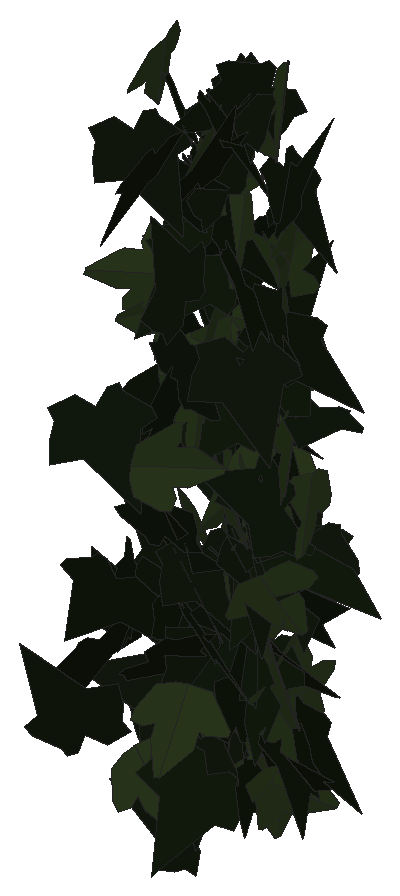
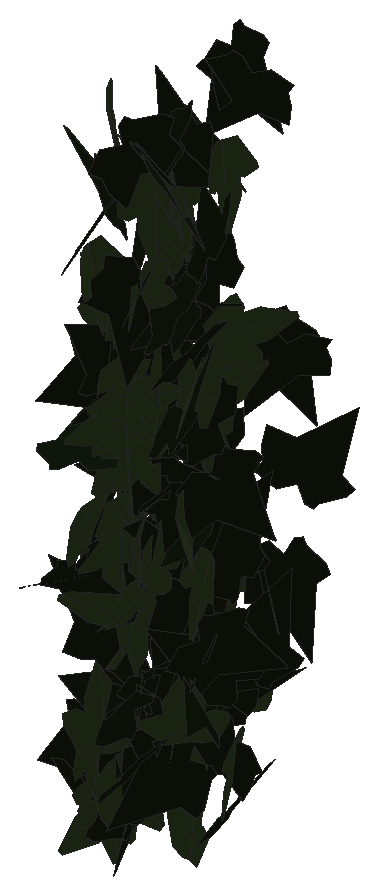
# SketchUp Ruby script. Lengths in inches.
U = 1.inch
M = Sketchup.active_model
def pt(a) = Geom::Point3d.new(a.map { |v| v * U })
def face(e, loops, mat)
  f = e.add_face(loops[0].map { |a| pt(a) })
  loops[1..].each { |l| e.add_face(l.map { |a| pt(a) }).erase! }
  f.material = f.back_material = mat if mat
  f
end
# faces: each face lists its corners as indices into pts; further lists are holes
def faces(e, pts, list, mat = nil) = list.each { |f| face(e, (f[0].is_a?(Array) ? f : [f]).map { |l| l.map { |i| pts[i] } }, mat) }
# xy, xz, yz: faces in a plane at the given z, y or x. An outline is a flat list of corners, or four numbers for a rectangle; further outlines are holes
def ring(l) = l.size == 4 ? [[l[0], l[1]], [l[2], l[1]], [l[2], l[3]], [l[0], l[3]]] : l.each_slice(2).to_a
def flat(e, list, mat, &to3) = list.each { |f| face(e, (f[0].is_a?(Array) ? f : [f]).map { |l| ring(l).map { |u, v| to3.(u, v) } }, mat) }
def xy(e, z, list, mat = nil) = flat(e, list, mat) { |x, y| [x, y, z] }
def xz(e, y, list, mat = nil) = flat(e, list, mat) { |x, z| [x, y, z] }
def yz(e, x, list, mat = nil) = flat(e, list, mat) { |y, z| [x, y, z] }
def lines(e, pts, list) = list.each { |a, b| e.add_line(pt(pts[a]), pt(pts[b])) }
# prism: a flat outline (further loops are holes) pulled along v
def prism(e, loops, v, mat = nil)
  f = face(e, loops, mat); d = Geom::Vector3d.new(v.map { |x| x * U })
  f.pushpull(f.normal.samedirection?(d) ? d.length : -d.length)
end
def box(e, o, s, mat = nil) = prism(e, [[o, [o[0] + s[0], o[1], o[2]], [o[0] + s[0], o[1] + s[1], o[2]], [o[0], o[1] + s[1], o[2]]]], [0, 0, s[2]], mat)
def at(x, y, z, deg = 0) = Geom::Transformation.translation(pt([x, y, z])) * Geom::Transformation.rotation(ORIGIN, Z_AXIS, deg.degrees)
def axes(o, x, y, z) = Geom::Transformation.new([*x, 0, *y, 0, *z, 0, *pt(o).to_a, 1])
def part(name) = M.definitions.add(name)
# library, detail: a bought-in or finely detailed component or shape, given as its bounding box
def library(name, o, s) = part(name).tap { |d| box(d.entities, o, s) }
def detail(e, o, s) = box(e.add_group.entities, o, s)
def put(e, d, t, mat = nil) = e.add_instance(d, t).tap { |i| i.material = mat if mat }
def group(e, t, mat = nil) = e.add_group.tap { |g| g.transformation = t; g.material = mat if mat }.entities
root = M.entities
M.materials.add("efeu1").color = [18, 25, 13]
M.materials.add("efeu2").color = [43, 57, 29]
c1 = part("ivyleaf_9")
p = [[1.54,2.16,1.25],[1.36,2.04,1.19],[-0.21,0.99,0.68],[-0.71,1.11,0.82],[-0.85,0.86,0.67],[-0.8,0.17,0.21],
  [-0.9,-0.01,0.1],[-0.67,-0.16,-0.02],[-0.08,-0.08,-0.05],[-0.03,-0.6,-0.4],[0.65,-0.88,-0.66],[0.83,-0.6,-0.49],
  [1.29,-0.42,-0.43],[1.8125,-0.07,-0.26],[1.21,0.44,0.15]]
faces(c1.entities,p,[[0,1,2,3,4,5,6,7,8,9,10,11,12,13,14]],"efeu1")
c2 = part("ivyleaf_10")
p = [[0,0.5,-0.03],[-0.0625,2.02,-0.43],[-0.19,2.01,-0.46],[-0.54,1.05,-0.29],[-0.52,0.625,-0.18],[-0.83,0.76,-0.28],
  [-1.16,0.64,-0.33],[-1.15,0.33,-0.24],[-0.77,-0.39,0.02],[-0.3,-0.51,0.16],[0.04,-0.48,0.23],[-0.02,2.01,-0.4375],
  [-0.06,2.01,-0.43],[0.04,-0.49,0.23],[0.67,-0.49,0.14],[1.38,0.36,-0.2],[1.375,0.51,-0.24],[0.81,0.65,-0.19],
  [0.62,0.59,-0.15],[0.6,1.09,-0.28],[0.5,1.23,-0.31]]
faces(c2.entities,p,[[0,1,2,3,4,5,6,7,8,9,10],[11,12,0,13,14,15,16,17,18,19,20]],"efeu2")
put(root,c1,axes([47.49,216.33,226.02],[0.21781,0.01885,0.44967],[-0.44525,0.0819,0.21224],[-0.06566,-0.49289,0.05246]))
put(root,c1,axes([47.89,216.47,228.31],[0.17503,0.16112,-0.43977],[-0.31626,-0.30562,-0.23785],[-0.34546,0.36143,-0.00507]))
put(root,c1,axes([47.26,218.06,233.63],[-0.22088,0.32793,-0.30606],[0.15027,-0.26735,-0.3949],[-0.42265,-0.26643,0.01955]))
put(root,c1,axes([47.9375,217.84,231.89],[-0.39914,0.08091,-0.29007],[-0.29244,0.01075,0.40541],[0.07185,0.49329,0.03874]))
put(root,c1,axes([46.18,218.26,229.4375],[-0.08221,-0.34357,-0.35383],[0.09276,0.34154,-0.35319],[0.48439,-0.12371,0.00758]))
put(root,c1,axes([47.67,218.6,224.39],[-0.26324,-0.41747,0.08016],[-0.04259,-0.06791,-0.49353],[0.42296,-0.26666,0.0002]))
put(root,c1,axes([46.23,218.23,226.06],[-0.06634,0.46022,-0.18384],[0.02921,-0.18153,-0.46497],[-0.49472,-0.07243,-0.0028]))
put(root,c2,axes([47.4,218.47,225.45],[0.3895,0.28688,-0.12645],[-0.1012,-0.07582,-0.48374],[-0.29673,0.40243,-0.001]))
put(root,c1,axes([46.66,218.45,233.61],[-0.17634,-0.19949,-0.42321],[0.27207,0.32422,-0.26619],[0.38063,-0.32417,-0.0058]))
put(root,c2,axes([47.07,218.26,228.9],[0.04644,0.0753,0.49211],[0.15113,0.46879,-0.08599],[-0.47435,0.15673,0.02078]))
put(root,c2,axes([46.58,218.71,224.16],[0.23616,0.38956,0.20609],[0.0978,0.18166,-0.45545],[-0.42973,0.25543,0.0096]))
put(root,c1,axes([46.2,218.9,226.49],[-0.08348,0.03463,-0.49176],[-0.48573,0.07947,0.08806],[0.08426,0.49243,0.02038]))
put(root,c1,axes([46.9,219.47,224.25],[0.019,-0.49426,0.0731],[0.00268,-0.07306,-0.49463],[0.49963,0.01919,-0.00013]))
put(root,c1,axes([47.54,219.61,231.16],[0.10194,-0.30953,0.37921],[0.10601,-0.36419,-0.32577],[0.47788,0.14682,-0.00863]))
put(root,c1,axes([46.9,219.48,232.57],[0.14254,0.41484,0.23998],[-0.08465,-0.22464,0.4386],[0.47172,-0.16567,0.00619]))
put(root,c1,axes([47.48,219.66,230.07],[-0.166,-0.35848,-0.3065],[0.12153,0.28144,-0.39499],[0.45571,-0.20563,-0.00631]))
put(root,c1,axes([46.34,219.78,229.3],[-0.01079,0.01661,0.49961],[0.37804,-0.32669,0.01902],[0.32707,0.37815,-0.00551]))
put(root,c1,axes([46.18,220.01,224.55],[-0.12882,-0.3893,-0.2861],[-0.06181,-0.28038,0.40935],[-0.47915,0.14084,0.02411]))
put(root,c1,axes([45.57,219.83,225.375],[0.35395,-0.03107,0.35179],[-0.34957,0.03992,0.35525],[-0.05016,-0.49743,0.00653]))
put(root,c1,axes([46.02,219.82,226.9],[0.31101,-0.17026,0.35254],[-0.30949,0.16881,0.35456],[-0.23976,-0.43876,-0.00038]))
put(root,c2,axes([45.76,220.08,230.52],[0.04849,0.11812,0.48342],[-0.17845,-0.44928,0.12768],[0.46455,-0.18492,-0.00142]))
put(root,c1,axes([46.17,220.07,222.48],[0.07866,-0.49061,-0.05583],[0.01855,-0.05356,0.49678],[-0.49342,-0.08023,0.00978]))
put(root,c1,axes([47.71,220.11,227.73],[0.06037,-0.47696,-0.13734],[0.01842,-0.13611,0.48077],[-0.496,-0.06311,0.00114]))
put(root,c1,axes([45.51,220.125,226.94],[0.0738,-0.17302,0.46327],[0.28137,-0.3705,-0.1832],[0.40667,0.28774,0.04268]))
put(root,c1,axes([46.04,219.5625,225.12],[0.29819,0.34852,0.19904],[0.11983,0.15934,-0.45853],[-0.38304,0.32116,0.0115]))
put(root,c1,axes([46.4375,219.83,225.82],[0.44516,-0.1573,-0.16459],[-0.1521,0.06348,-0.47205],[0.16941,0.47035,0.00867]))
put(root,c1,axes([46.66,220.07,233.27],[0.40605,-0.28771,-0.04842],[-0.03939,0.02815,-0.49765],[0.28909,0.40796,0.0002]))
put(root,c1,axes([45.97,219.72,228.53],[0.05912,0.08961,0.48834],[0.184,0.45282,-0.10537],[-0.46114,0.19217,0.02056]))
put(root,c2,axes([45.72,219.93,224.04],[-0.24624,0.38847,0.1961],[-0.13263,0.1476,-0.45894],[-0.41446,-0.27803,0.03035]))
put(root,c1,axes([46.47,220.08,226.625],[-0.14816,-0.21296,-0.42743],[0.2465,0.34919,-0.25943],[0.40901,-0.2876,0.00151]))
put(root,c1,axes([46.28,220.47,230.77],[-0.34095,-0.3342,0.14853],[-0.09063,-0.11952,-0.47697],[0.35431,-0.35217,0.02092]))
put(root,c1,axes([45.63,220.15,224.26],[-0.04649,-0.0741,-0.49229],[0.43762,0.22962,-0.07589],[0.23733,-0.43793,0.0435]))
put(root,c2,axes([46.1875,220.3125,228.78],[0.37505,-0.23154,0.23606],[0.19539,-0.13279,-0.44067],[0.26676,0.4228,-0.00913]))
put(root,c2,axes([46.9,220.28,231.77],[0.41754,-0.22586,0.15701],[0.14097,-0.06938,-0.47467],[0.2362,0.44065,0.00573]))
put(root,c2,axes([45.71,220.53,229.79],[-0.07086,-0.06146,-0.49112],[-0.21945,-0.4408,0.08682],[-0.44364,0.22786,0.0355]))
put(root,c2,axes([46.07,220.54,222.7],[0.02981,-0.36176,-0.34386],[0.05299,-0.34023,0.36254],[-0.49629,-0.05806,0.01806]))
put(root,c2,axes([47.51,220.13,226.51],[-0.3098,-0.3242,-0.22118],[0.1502,0.16239,-0.44841],[0.36258,-0.34427,-0.00323]))
put(root,c1,axes([45.66,220.43,231.62],[0.05134,-0.05819,0.49394],[0.34895,-0.34962,-0.07746],[0.3544,0.35268,0.00471]))
put(root,c2,axes([46.44,220.27,232.73],[0.13584,-0.46576,-0.12089],[-0.04109,0.11393,-0.48511],[0.47944,0.14173,-0.00732]))
put(root,c1,axes([46.89,220.04,232.16],[-0.40687,0.14485,-0.25195],[-0.23758,0.08386,0.43188],[0.16738,0.47115,0.00059]))
put(root,c1,axes([46.35,220.63,223.98],[-0.02483,-0.03502,0.49815],[0.03693,-0.49753,-0.03313],[0.49802,0.03515,0.02729]))
put(root,c1,axes([46.875,220.46,225.64],[0.27275,-0.01645,0.41873],[-0.41857,0.01327,0.27317],[-0.0201,-0.49955,-0.00653]))
put(root,c1,axes([46.9,220.62,226.48],[0.10114,-0.46401,0.1564],[0.03289,-0.15291,-0.47491],[0.48856,0.10635,-0.00041]))
put(root,c1,axes([47.67,220.19,232.04],[-0.18853,0.42887,0.17471],[0.0613,-0.16387,0.46839],[0.45902,0.19803,0.00921]))
put(root,c2,axes([46.83,220.32,227.03],[-0.39447,0.27374,-0.13952],[-0.11644,0.07692,0.48013],[0.28432,0.41128,0.00306]))
put(root,c1,axes([46.38,220.15,224.8],[-0.17488,-0.16186,0.43956],[0.31542,0.30619,0.23824],[-0.3463,0.36063,-0.00498]))
put(root,c1,axes([45.55,220.62,228.66],[-0.04787,0.21794,-0.44745],[0.09559,-0.43712,-0.22314],[-0.48844,-0.1069,0.00018]))
put(root,c1,axes([45.81,220.7,225.67],[0.1499,-0.26808,0.39455],[0.18428,-0.34891,-0.30708],[0.43997,0.23748,-0.0058]))
put(root,c2,axes([47.34,220.625,233.66],[0.30559,-0.28377,0.27584],[0.2242,-0.16305,-0.41611],[0.32611,0.37801,0.02759]))
put(root,c1,axes([46.75,220.26,231.59],[0.29195,-0.20327,-0.35134],[-0.25355,0.24663,-0.35339],[0.31698,0.38451,0.04093]))
put(root,c1,axes([45.625,220.78,226.09],[-0.01746,-0.02202,-0.49921],[0.0355,-0.49831,0.02074],[-0.49843,-0.03472,0.01897]))
put(root,c1,axes([46.88,220.24,224.24],[-0.04955,-0.21607,0.44817],[0.13947,0.4263,0.22094],[-0.47759,0.14691,0.01803]))
put(root,c1,axes([45.53,220.25,225.32],[-0.03331,-0.00593,0.49885],[0.48838,0.10171,0.03381],[-0.10188,0.48951,-0.00098]))
put(root,c2,axes([45.5,220.4375,233.58],[0.04498,-0.48627,-0.10732],[-0.00764,0.10707,-0.48834],[0.49791,0.04557,0.0022]))
put(root,c2,axes([45.78,220.43,228.89],[0.06463,-0.00647,-0.49576],[0.49532,-0.02135,0.06485],[-0.02201,-0.4995,0.00365]))
put(root,c1,axes([47.2,220.75,226.67],[-0.30978,-0.39217,0.01543],[-0.00887,-0.01265,-0.49976],[0.39237,-0.30991,0.00088]))
put(root,c2,axes([46.31,220.53,231.99],[-0.19082,0.00161,0.46215],[0.46215,0.00348,0.1908],[-0.0026,0.49999,-0.00282]))
put(root,c2,axes([47.63,220.4,224.58],[-0.354,0.2784,-0.2172],[-0.16901,0.13644,0.45035],[0.31003,0.39227,-0.0025]))
put(root,c1,axes([46.99,220.75,233.375],[-0.10476,0.04276,-0.48703],[-0.11521,-0.48622,-0.0179],[-0.47513,0.10847,0.11172]))
put(root,c1,axes([46.87,220.64,233.27],[-0.48671,0.05054,-0.10277],[0.10153,-0.01723,-0.48928],[-0.053,-0.49714,0.00651]))
put(root,c2,axes([47.33,220.78,228.35],[0.14114,-0.32184,0.35566],[0.27305,-0.2509,-0.3354],[0.39436,0.28891,0.10494]))
put(root,c1,axes([45.58,220.58,229.47],[0.31215,-0.14059,0.36441],[0.32209,-0.17124,-0.34196],[0.22096,0.44823,-0.01634]))
put(root,c1,axes([46.78,220.95,224.86],[-0.22935,-0.28278,0.34268],[-0.21303,-0.26844,-0.36409],[0.38989,-0.31301,0.00265]))
put(root,c2,axes([46.37,220.93,227.15],[-0.01369,0.00858,0.49974],[0.19375,-0.46075,0.01322],[0.46073,0.19401,0.00929]))
put(root,c2,axes([45.87,220.47,227.01],[-0.41185,0.26964,0.08762],[-0.0781,0.04064,-0.49219],[-0.27255,-0.4191,0.00864]))
put(root,c2,axes([45.99,220.55,223.66],[-0.01022,-0.00912,0.49981],[0.4865,0.11477,0.01204],[-0.11494,0.48657,0.00653]))
put(root,c1,axes([45.94,220.61,228.24],[-0.0763,-0.39108,-0.30205],[0.04722,0.29846,-0.39836],[0.49188,-0.08932,-0.00861]))
put(root,c2,axes([46.74,220.67,229.7],[-0.34038,-0.33969,0.13693],[-0.09482,-0.09882,-0.48088],[0.35376,-0.35333,0.00285]))
put(root,c1,axes([45.66,220.65,227.94],[0.38564,-0.31706,-0.0275],[-0.02079,0.01801,-0.49924],[0.31757,0.3862,0.00071]))
put(root,c1,axes([46.36,220.89,228.57],[-0.44764,-0.22243,0.01207],[-0.00905,-0.00891,-0.49984],[0.22258,-0.44771,0.00395]))
put(root,c2,axes([46.79,220.8,225.49],[-0.21524,0.0705,0.44576],[0.42685,-0.12855,0.22644],[0.14654,0.47802,-0.00485]))
put(root,c1,axes([46.61,220.5,233.01],[-0.2934,0.34808,0.20678],[-0.1346,0.15698,-0.45524],[-0.38183,-0.3228,0.00158]))
put(root,c1,axes([47.16,220.97,223.58],[0.142,-0.40859,0.25077],[0.08468,-0.23605,-0.43256],[0.47187,0.16532,0.00216]))
put(root,c2,axes([47.03,220.86,230.64],[-0.30158,0.11046,0.38321],[0.34851,-0.16055,0.32056],[0.19387,0.46046,0.01984]))
put(root,c1,axes([47.35,220.71,232.29],[0.28238,-0.37576,-0.17048],[-0.09566,0.14134,-0.46997],[0.40138,0.29804,0.00793]))
put(root,c1,axes([46.85,220.48,223.45],[0.17869,-0.12424,-0.45015],[-0.36044,0.26975,-0.21753],[0.29691,0.40224,0.00684]))
put(root,c1,axes([45.3125,221.06,232.44],[0.02071,-0.20478,0.45567],[0.1527,-0.43164,-0.20092],[0.47566,0.14749,0.04466]))
put(root,c1,axes([46.28,220.68,230.25],[0.00077,-0.02316,-0.49946],[0.40779,0.28903,-0.01277],[0.28932,-0.40734,0.01933]))
put(root,c1,axes([46.84,220.89,224.96],[-0.3471,-0.19459,-0.30274],[0.29014,0.09755,-0.39535],[0.21293,-0.45013,0.0452]))
put(root,c2,axes([46.4375,220.59,230.16],[0.06558,-0.41322,-0.27376],[-0.0167,0.27415,-0.41781],[0.4954,0.06395,0.02215]))
put(root,c2,axes([46.85,220.37,226.36],[-0.01803,0.07385,0.49419],[-0.11349,0.48098,-0.07601],[-0.48662,-0.11491,-0.00059]))
put(root,c1,axes([46.39,220.78,228.54],[0.36469,-0.17537,0.29367],[0.27909,-0.09562,-0.40369],[0.19775,0.45837,0.02814]))
put(root,c1,axes([47.16,220.83,225.86],[0.40197,0.06868,-0.28931],[0.27527,0.09801,0.40573],[0.11245,-0.48547,0.04098]))
put(root,c2,axes([46.56,220.72,232.79],[-0.48165,0.00372,0.13417],[-0.13416,0.00171,-0.48166],[-0.00404,-0.49998,-0.00065]))
put(root,c1,axes([46.96,220.58,227.01],[0.03298,-0.0524,0.49615],[-0.19195,0.45763,0.06109],[-0.46051,-0.1945,0.01007]))
put(root,c2,axes([46.86,221.07,223.63],[-0.12164,-0.38326,0.29718],[-0.08483,-0.28485,-0.40208],[0.4775,-0.14823,0.00427]))
put(root,c1,axes([46.91,221.07,227.375],[-0.13502,-0.48075,-0.02539],[0.00867,0.02394,-0.49935],[0.48135,-0.13529,0.00187]))
put(root,c2,axes([47.06,220.84,230.71],[-0.39667,-0.12661,0.27681],[0.26216,0.08895,0.41636],[-0.15468,0.47545,-0.00419]))
put(root,c2,axes([47.18,220.88,223.24],[-0.19377,-0.46054,0.0189],[-0.00859,-0.01689,-0.49964],[0.46085,-0.19395,-0.00137]))
put(root,c1,axes([47.14,221.22,227.51],[-0.08159,-0.07649,0.48733],[-0.06552,-0.4879,-0.08755],[0.48893,-0.07814,0.06959]))
put(root,c1,axes([46.8,220.64,231.27],[0.21238,0.44196,-0.0978],[-0.04342,-0.08764,-0.49034],[-0.45057,0.21677,0.00115]))
put(root,c2,axes([45.91,220.74,224.59],[0.40029,0.2953,-0.0507],[0.03568,0.03703,0.49735],[0.29749,-0.40178,0.00858]))
put(root,c2,axes([46.97,220.67,225.96],[-0.0806,-0.12723,0.47678],[0.36069,0.31449,0.1449],[-0.33675,0.3673,0.04109]))
put(root,c1,axes([45.91,220.52,225.22],[-0.23987,0.15073,-0.412],[-0.34865,0.21952,0.28329],[0.26628,0.42319,-0.00021]))
put(root,c1,axes([47.22,220.6,229.86],[-0.09485,-0.08561,0.4834],[0.33068,0.35274,0.12735],[-0.36284,0.34386,-0.01029]))
put(root,c1,axes([47.4,221.26,228.58],[-0.23564,-0.40932,0.16411],[0.32453,-0.28694,-0.24968],[0.29858,-0.01115,0.40091]))
put(root,c1,axes([47.17,220.81,229.78],[0.00064,-0.03314,-0.4989],[0.38051,0.32368,-0.02101],[0.32436,-0.37965,0.02563]))
put(root,c1,axes([45.625,221.11,230.78],[0.08413,-0.49237,0.02232],[0.00478,-0.02182,-0.4995],[0.49285,0.08426,0.00103]))
put(root,c2,axes([46.58,220.73,231.22],[-0.03763,0.02676,-0.49786],[-0.40744,0.28611,0.04617],[0.28736,0.40918,0.00027]))
put(root,c2,axes([47.41,221.06,227.47],[-0.02475,-0.48757,0.10802],[0.12192,-0.11078,-0.47209],[0.48428,0.00297,0.12437]))
put(root,c2,axes([47.39,220.97,231.53],[0.10169,-0.48806,-0.03812],[-0.00647,0.03759,-0.49854],[0.48951,0.10189,0.00133]))
put(root,c2,axes([46.89,221.04,227.85],[0.29784,0.35322,-0.19112],[-0.11557,-0.1525,-0.46194],[-0.38462,0.31935,-0.0092]))
put(root,c1,axes([47.32,220.97,224.02],[-0.01697,-0.01044,-0.4996],[0.46484,0.18314,-0.01962],[0.1834,-0.46514,0.00349]))
put(root,c2,axes([46.96,220.99,229.56],[-0.16234,0.03188,-0.47184],[-0.47253,0.00921,0.1632],[0.0191,0.4989,0.02714]))
put(root,c1,axes([46.75,221.03,223.2],[0.18516,-0.18498,0.42602],[0.39284,-0.1823,-0.24989],[0.24778,0.42726,0.07783]))
put(root,c1,axes([46.92,221.01,229.63],[0.05618,-0.45456,-0.20054],[-0.00733,0.20104,-0.45774],[0.49678,0.05438,0.01592]))
put(root,c1,axes([47.32,220.94,226.67],[0.23734,-0.40419,-0.17407],[0.21162,0.27823,-0.3575],[0.38586,0.09603,0.30314]))
put(root,c1,axes([47.39,221.1,226.71],[-0.27753,-0.35193,-0.22164],[0.13011,0.17962,-0.44812],[0.39503,-0.3064,-0.00812]))
put(root,c1,axes([46.65,221.07,224.83],[0.25718,-0.22283,0.36634],[0.32334,-0.17979,-0.33634],[0.28162,0.40991,0.05162]))
put(root,c2,axes([46.79,220.64,227.31],[-0.04855,0.15809,-0.47186],[-0.14377,0.44942,0.16537],[0.47642,0.15174,0.00182]))
put(root,c2,axes([47.25,221.09,224.16],[-0.02455,-0.49533,0.06358],[0.12079,-0.06765,-0.48045],[0.48457,-0.00823,0.12298]))
put(root,c2,axes([46.86,221.03,227.37],[0.1136,0.47941,-0.0852],[-0.01514,-0.08397,-0.49267],[-0.48669,0.11451,-0.00456]))
put(root,c2,axes([46.7,220.66,229.68],[0.01726,-0.04389,-0.49777],[0.21536,0.45009,-0.03222],[0.45091,-0.21329,0.03444]))
put(root,c2,axes([46.98,221.01,229.14],[0.29341,0.40467,-0.01234],[-0.00896,-0.00874,-0.49984],[-0.40476,0.29354,0.00212]))
put(root,c1,axes([45.7,221.28,231.41],[0.18478,-0.36454,0.28804],[0.14707,-0.24815,-0.4084],[0.44071,0.23565,0.01552]))
put(root,c1,axes([45.625,221.03,231.55],[0.43078,-0.25351,0.01253],[0.00956,-0.00846,-0.49984],[0.25364,0.43088,-0.00244]))
put(root,c1,axes([45.76,221.33,229.49],[0.30194,-0.39743,-0.02973],[0.02756,-0.01639,0.49897],[-0.39759,-0.30295,0.01201]))
put(root,c2,axes([45.66,221.07,230.2],[-0.27929,0.38308,-0.15889],[0.09639,-0.12636,-0.47407],[-0.40337,-0.29544,-0.00326]))
put(root,c1,axes([47.09,221.04,223.32],[0.14724,-0.14931,0.4539],[-0.34371,0.29686,0.20914],[-0.33194,-0.37361,-0.01522]))
put(root,c2,axes([46.65,221.02,228.92],[-0.4382,-0.01446,-0.24036],[0.24075,-0.01668,-0.43791],[0.00465,-0.49951,0.02158]))
put(root,c2,axes([47.06,221.18,224.32],[-0.17834,-0.46251,-0.06539],[-0.00985,-0.06625,0.49549],[-0.46701,0.17802,0.01452]))
put(root,c2,axes([45.54,221.31,228.19],[0.24279,-0.29955,0.31831],[0.21924,-0.23155,-0.38512],[0.37813,0.32658,0.01891]))
put(root,c1,axes([45.95,220.73,224.0625],[0.32718,0.31438,0.21003],[0.15287,0.14404,-0.45374],[-0.3458,0.36113,-0.00187]))
put(root,c2,axes([46.94,220.84,228.61],[-0.18084,0.17238,0.43311],[-0.3733,0.22468,-0.24529],[-0.27918,-0.41208,0.04743]))
put(root,c1,axes([46.48,221.47,223.96],[-0.13104,-0.39104,0.28269],[-0.01363,-0.28981,-0.40721],[0.48233,-0.11443,0.0653]))
put(root,c2,axes([47.17,220.85,223.125],[-0.173,-0.26046,-0.39017],[0.20256,0.33362,-0.31252],[0.42313,-0.2662,-0.00992]))
